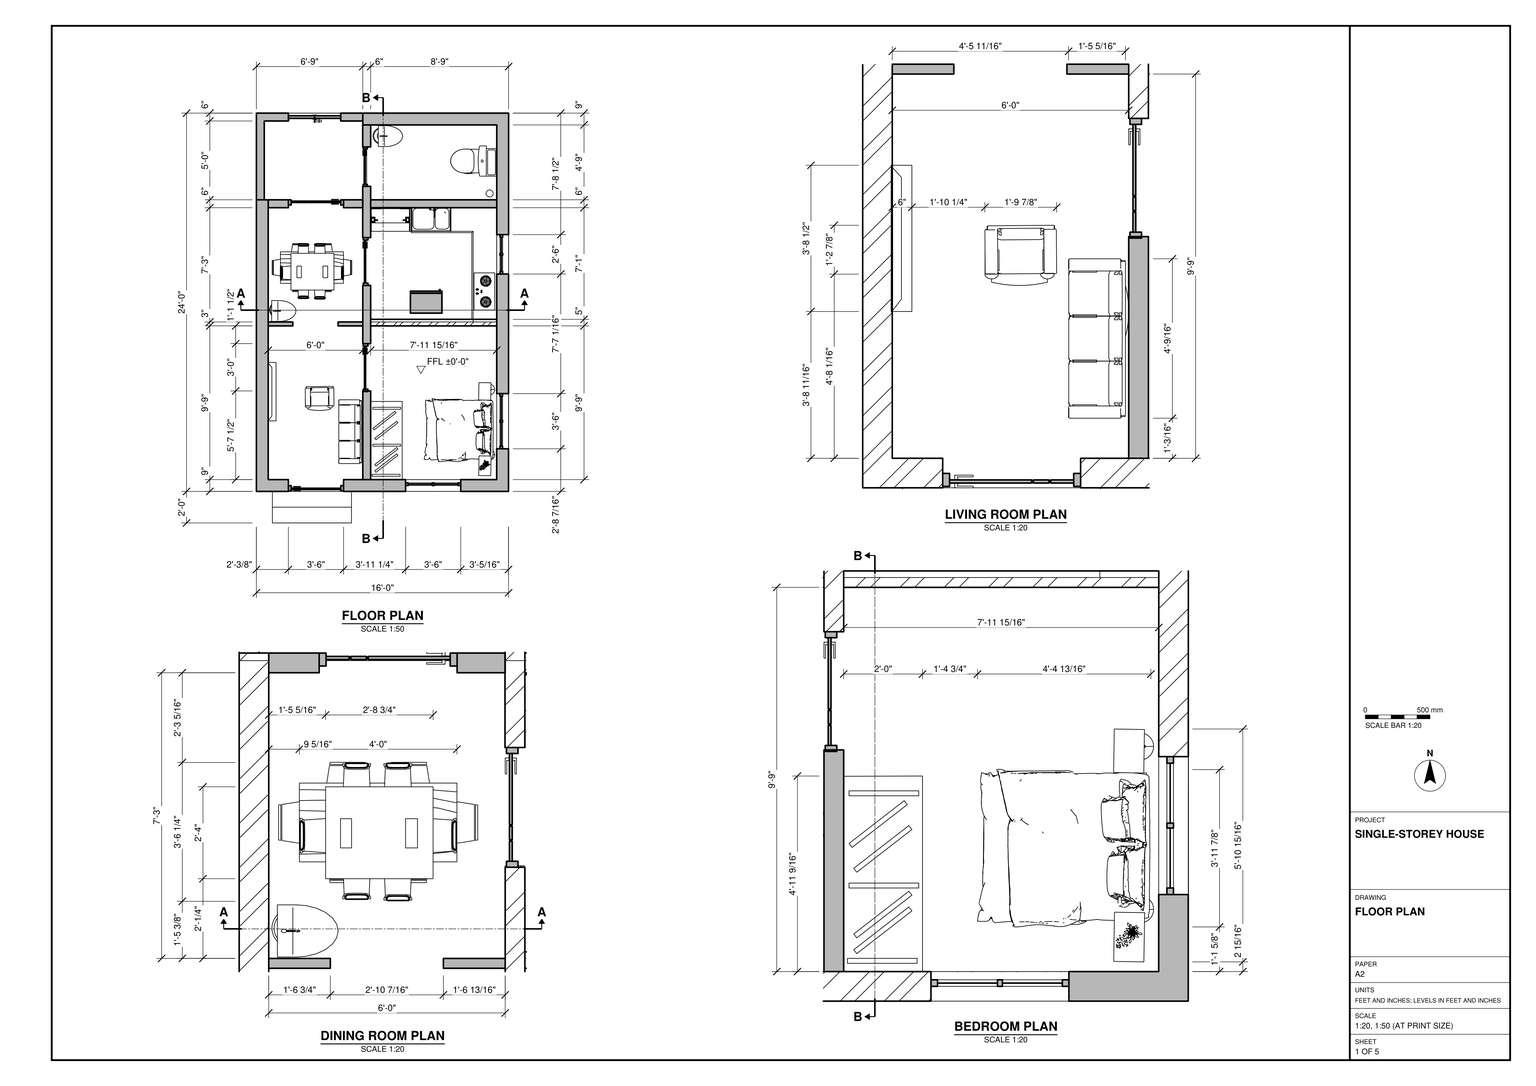
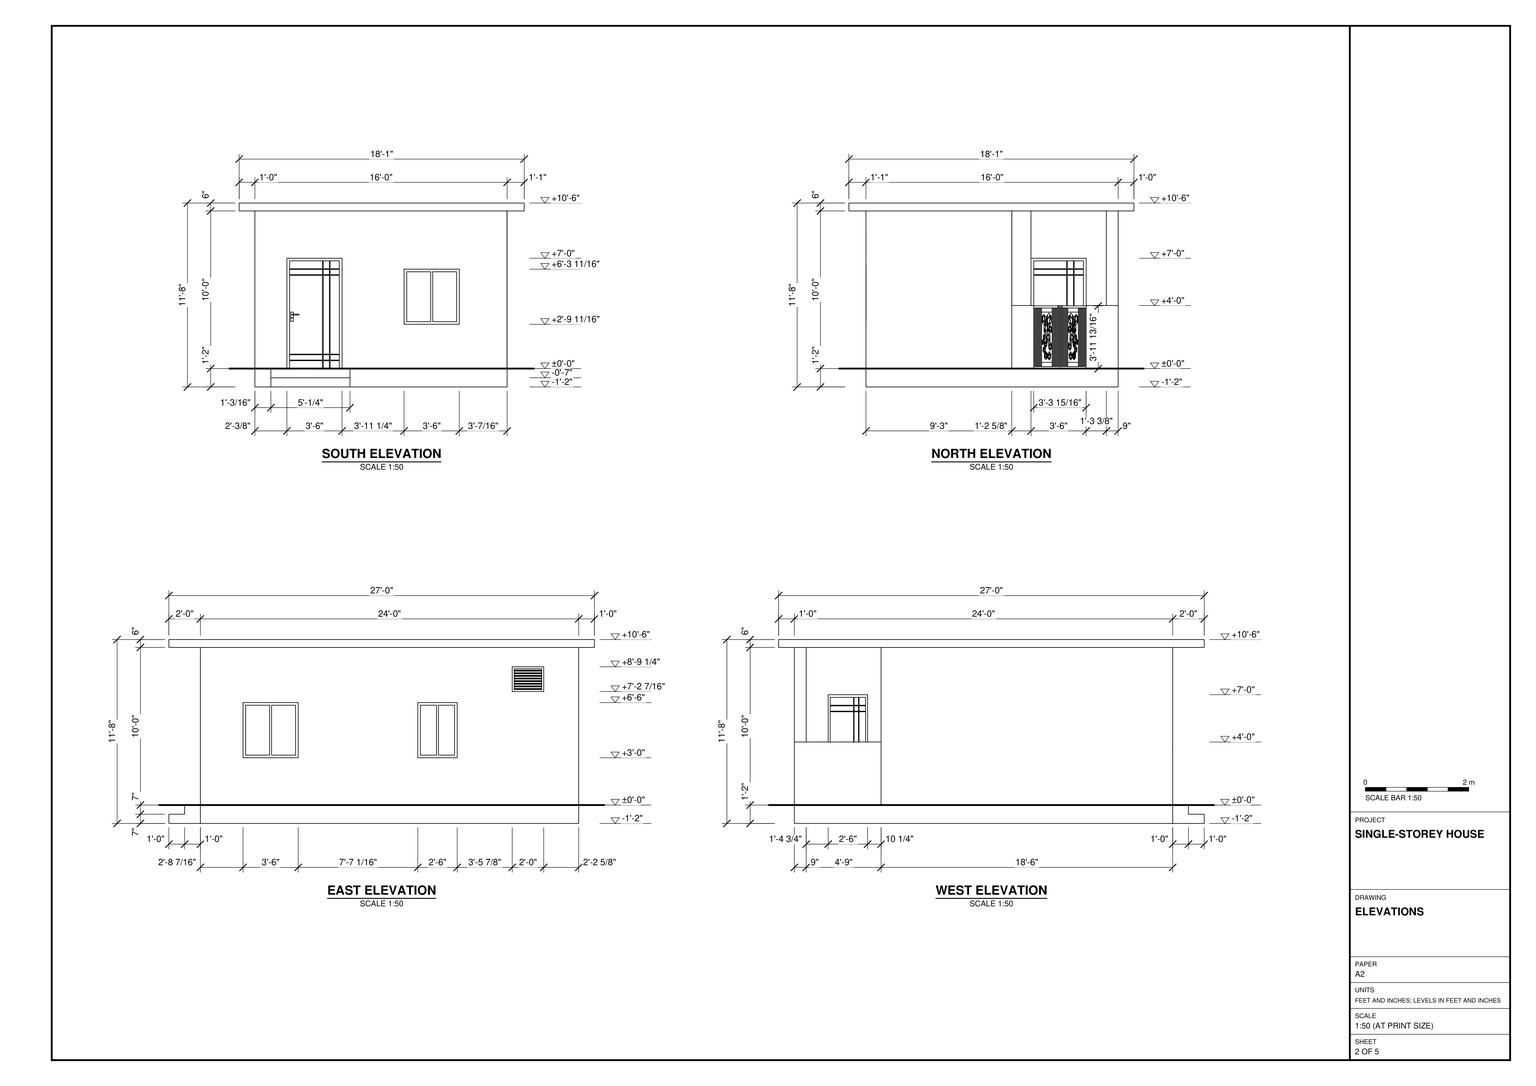
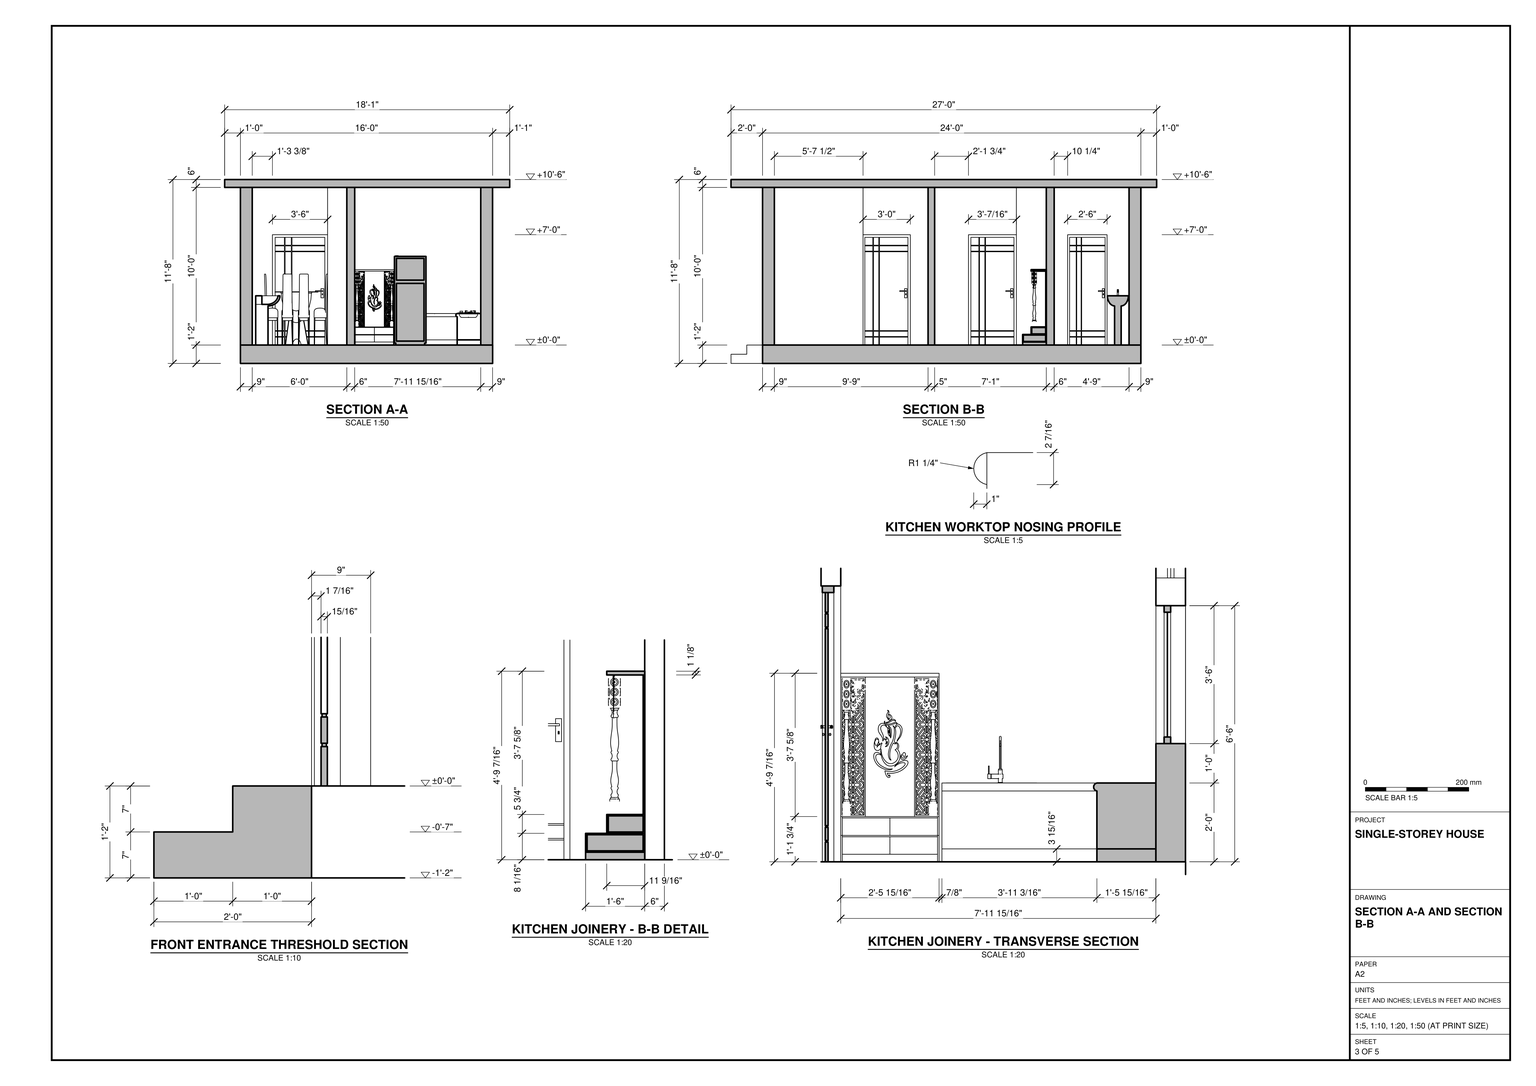
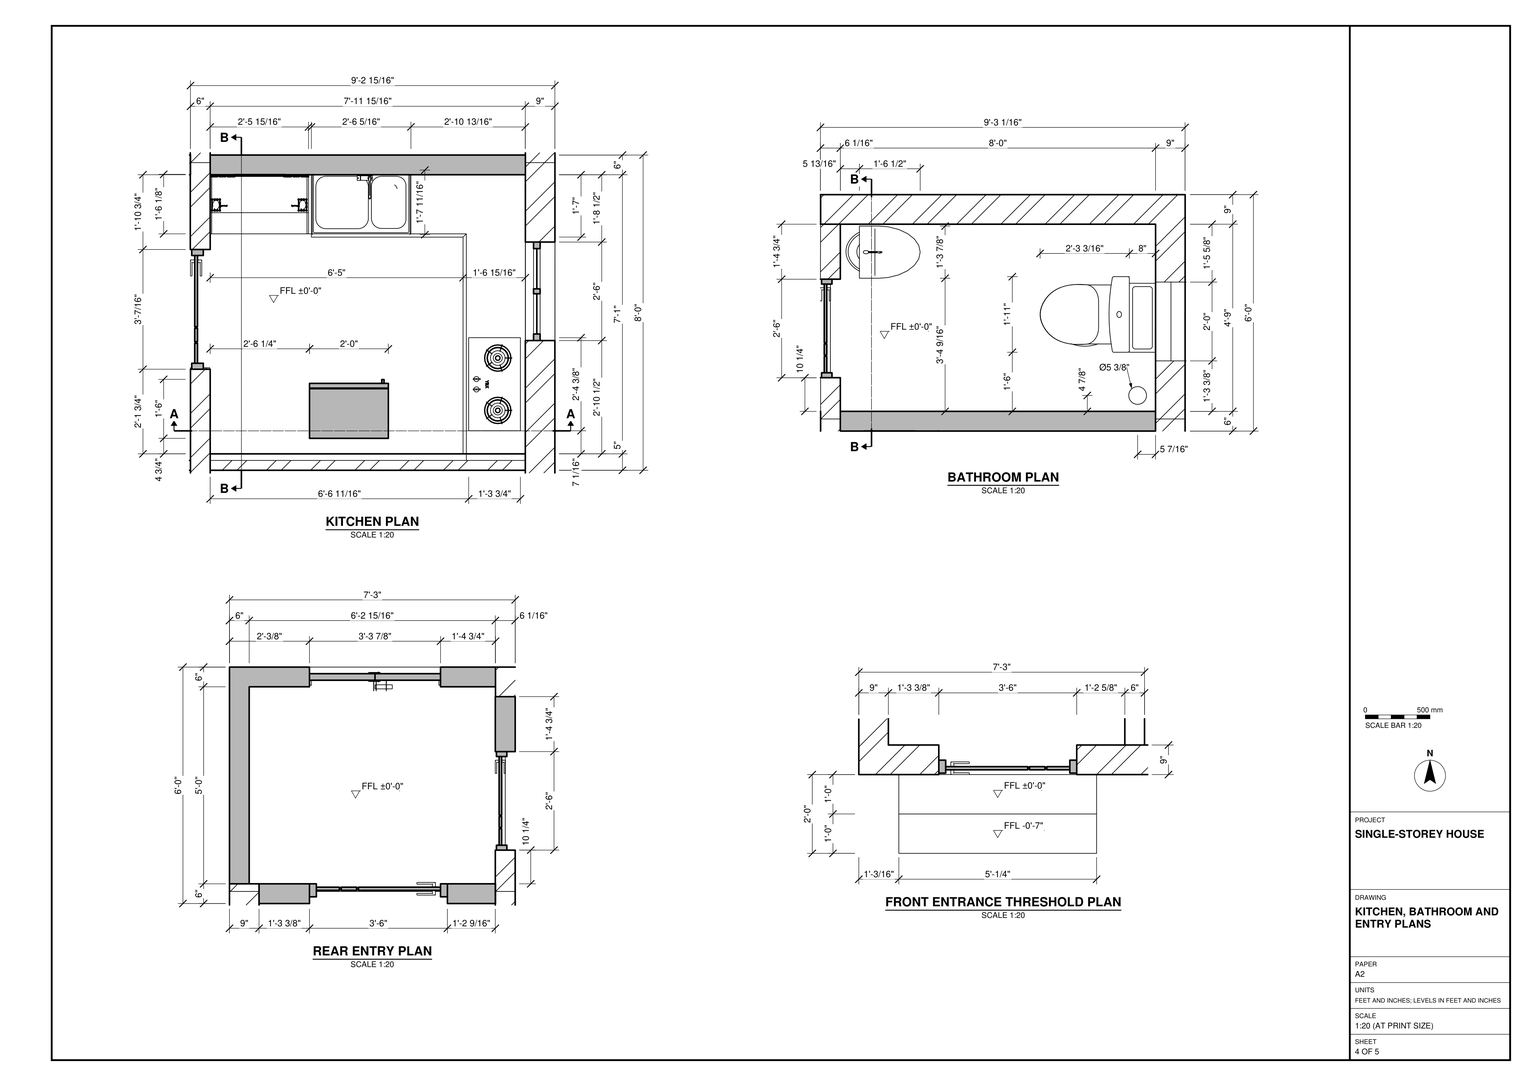
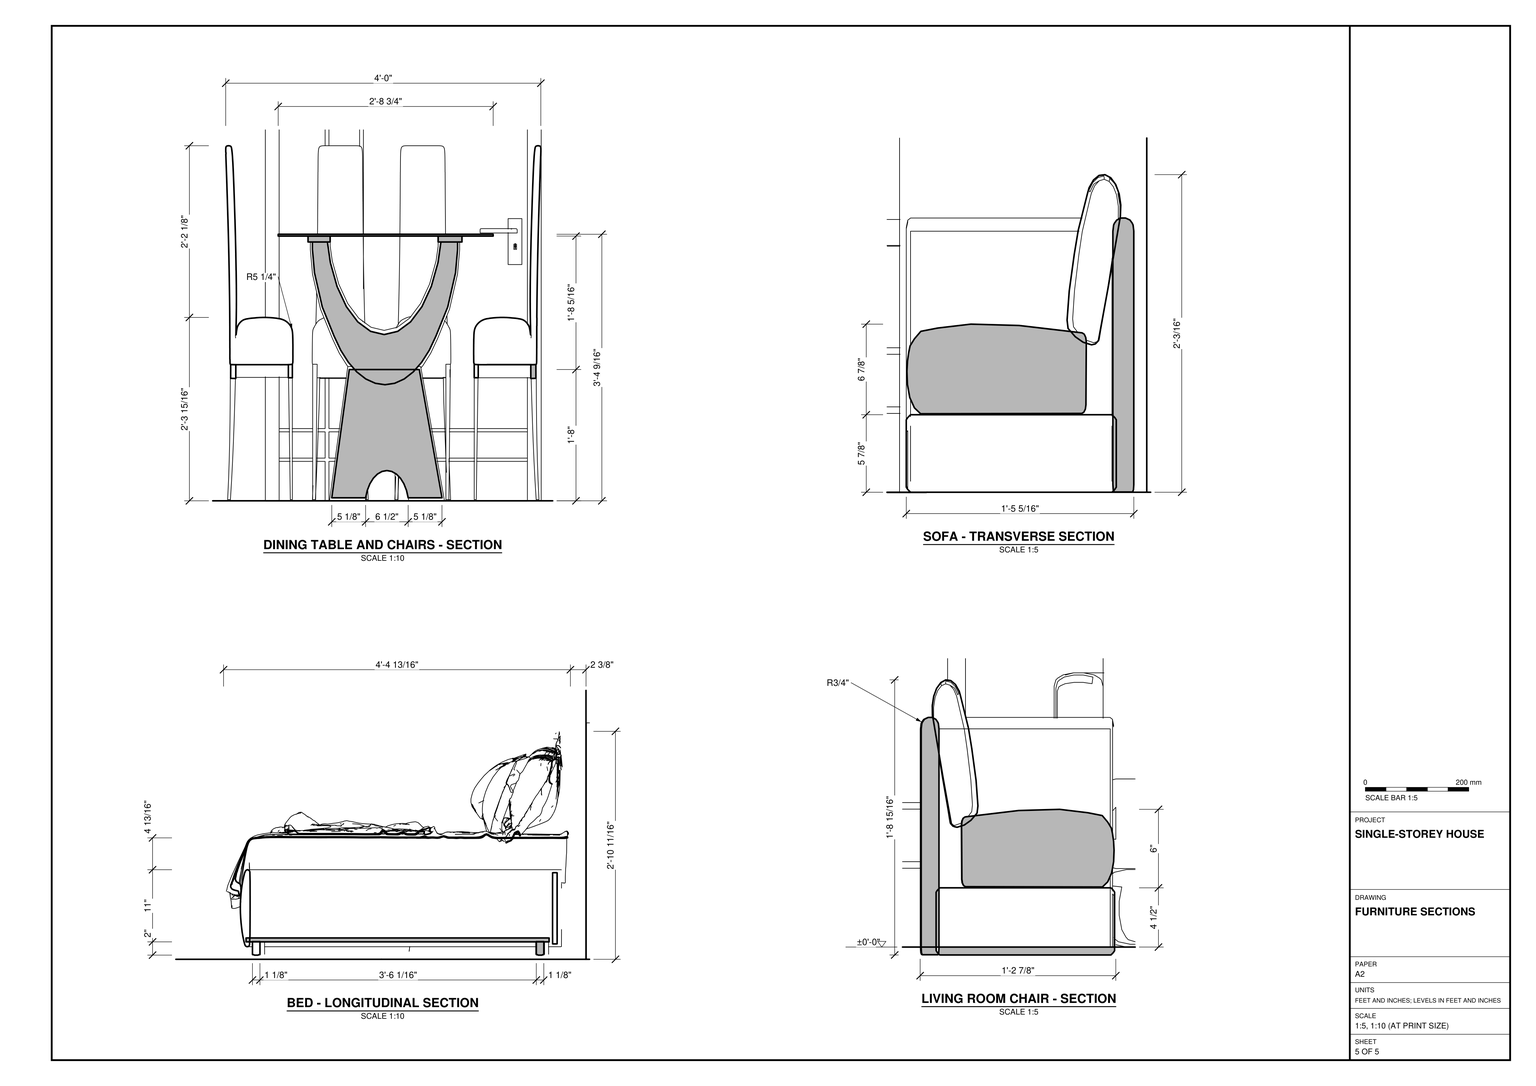
Build the single-storey house shown in task_files/diagram_01.pdf. Work in feet and inches. Set the finished ground floor at ±0'-0". The overall model is 18'-1" wide, 27'-0" long and 11'-8" high, including the raised base and projecting roof. The wall footprint is 16'-0" by 24'-0"; use this footprint, rather than the roof outline, to set out the rooms.

Model the floor slab, the stepped threshold at the south entrance and the flat roof slab with its unequal overhangs. Follow the plans and sections for wall thicknesses and door positions. Include the recessed area at the northwest corner, the framed windows and the high vent on the east elevation.

Place the living room and dining room along the west side. Arrange the sofa, chair and opposing wall unit as shown in the living room detail, and fit the dining table and chairs in the adjoining room. On the east side, model the bedroom with its bed, bedside units and storage, the kitchen with its fitted worktop and tall joinery unit, and the bathroom with its fixtures. Use the kitchen sections to shape the worktop edge and the base of the tall unit. Decor and loose items, including appliances, may be any suitable library components.

Keep the walls, slabs and roof as separate groups or components, and group each furniture or joinery piece separately. Use components for repeated parts. Save one SketchUp model as output_files/furnished_single_storey_house_with_a_stepped_entrance.skp.

# SketchUp Ruby script. Lengths in inches.
U = 1.inch
M = Sketchup.active_model
def pt(a) = Geom::Point3d.new(a.map { |v| v * U })
def face(e, loops, mat)
  f = e.add_face(loops[0].map { |a| pt(a) })
  loops[1..].each { |l| e.add_face(l.map { |a| pt(a) }).erase! }
  f.material = f.back_material = mat if mat
  f
end
# faces: each face lists its corners as indices into pts; further lists are holes
def faces(e, pts, list, mat = nil) = list.each { |f| face(e, (f[0].is_a?(Array) ? f : [f]).map { |l| l.map { |i| pts[i] } }, mat) }
# xy, xz, yz: faces in a plane at the given z, y or x. An outline is a flat list of corners, or four numbers for a rectangle; further outlines are holes
def ring(l) = l.size == 4 ? [[l[0], l[1]], [l[2], l[1]], [l[2], l[3]], [l[0], l[3]]] : l.each_slice(2).to_a
def flat(e, list, mat, &to3) = list.each { |f| face(e, (f[0].is_a?(Array) ? f : [f]).map { |l| ring(l).map { |u, v| to3.(u, v) } }, mat) }
def xy(e, z, list, mat = nil) = flat(e, list, mat) { |x, y| [x, y, z] }
def xz(e, y, list, mat = nil) = flat(e, list, mat) { |x, z| [x, y, z] }
def yz(e, x, list, mat = nil) = flat(e, list, mat) { |y, z| [x, y, z] }
def lines(e, pts, list) = list.each { |a, b| e.add_line(pt(pts[a]), pt(pts[b])) }
# prism: a flat outline (further loops are holes) pulled along v
def prism(e, loops, v, mat = nil)
  f = face(e, loops, mat); d = Geom::Vector3d.new(v.map { |x| x * U })
  f.pushpull(f.normal.samedirection?(d) ? d.length : -d.length)
end
def box(e, o, s, mat = nil) = prism(e, [[o, [o[0] + s[0], o[1], o[2]], [o[0] + s[0], o[1] + s[1], o[2]], [o[0], o[1] + s[1], o[2]]]], [0, 0, s[2]], mat)
def at(x, y, z, deg = 0) = Geom::Transformation.translation(pt([x, y, z])) * Geom::Transformation.rotation(ORIGIN, Z_AXIS, deg.degrees)
def axes(o, x, y, z) = Geom::Transformation.new([*x, 0, *y, 0, *z, 0, *pt(o).to_a, 1])
def part(name) = M.definitions.add(name)
# library, detail: a bought-in or finely detailed component or shape, given as its bounding box
def library(name, o, s) = part(name).tap { |d| box(d.entities, o, s) }
def detail(e, o, s) = box(e.add_group.entities, o, s)
def put(e, d, t, mat = nil) = e.add_instance(d, t).tap { |i| i.material = mat if mat }
def group(e, t, mat = nil) = e.add_group.tap { |g| g.transformation = t; g.material = mat if mat }.entities
root = M.entities
M.materials.add("0201 AP 9425 OUTDOOR PINK").color = [235, 192, 222]
M.materials.add("0241 AP 9602 Catmint Blossom-N").color = [202, 177, 218]
M.materials.add("0836 AP 7769 GREEN GLADE").color = [230, 225, 175]
M.materials.add("Colors In Model-1").color = [247, 231, 213]
M.materials.add("Picture1").color = [191, 175, 175]
M.materials.add("Picture2").color = [185, 162, 149]
M.materials.add("[Blacktop Old 02]").color = [143, 145, 145]
M.materials.add("[Carrera Marble]").color = [207, 207, 207]
M.materials.add("[Color B03]").color = [255, 140, 101]
M.materials.add("[Color H06]").color = [0, 204, 204]
M.materials.add("[Color L03]").color = [255, 101, 178]
M.materials.add("[Color M00]").color = [255, 255, 255]
M.materials.add("[Color M08]").color = [30, 30, 30]
M.materials.add("[Concrete Pavers Block Multi]").color = [124, 140, 145]
M.materials.add("[Field Rectangle Tile]").color = [196, 189, 179]
M.materials.add("[Formica Beige]").color = [211, 187, 149]
M.materials.add("[Marble Carrara Gold Floor Tile]").color = [225, 223, 217]
M.materials.add("[Metal Corrugated Shiny]1").color = [193, 193, 193]
M.materials.add("[Tile Border Travertine]").color = [160, 142, 112]
M.materials.add("[Translucent Glass Blue]").color = [100, 149, 237]
M.materials["[Translucent Glass Blue]"].alpha = 0.5
M.materials.add("[Wood Cherry Original]").color = [152, 86, 42]
M.materials.add("ft").color = [182, 168, 149]
c1 = library("Untitled",[0,0,0],[36,4.39,84])
c2 = library("Bedroom furniture set",[0,-4.61,0],[113.04,95.21,38.625])
c3 = part("Folded newspaper")
xy(c3.entities,0,[[0,2.76,135.04,80.9]],"Picture2")
xy(c3.entities,0.6,[[0,2.76,135.04,79.92]],"Colors In Model-1")
xy(c3.entities,1.45,[[0,2.8,135.04,79.875]],"Picture1")
xy(c3.entities,2.97,[[0,2.76,135.04,79.875]],"Colors In Model-1")
xy(c3.entities,3.82,[[0,2.76,135.04,79.92]],"Picture1")
xy(c3.entities,6.19,[[0,2.8,135.04,79.92]],"Picture1")
xy(c3.entities,7.04,[[0,2.04,135.04,2.76]],"Colors In Model-1")
xy(c3.entities,7.04,[[0,2.76,135.04,79.92],[0,79.92,24.36,80.26,127.45,80.26,135.04,79.92]],"Picture1")
xz(c3.entities,2.76,[[0,2.97,135.04,3.82]],"ft")
xz(c3.entities,79.92,[[0,6.19,135.04,7.04]],"Picture1")
yz(c3.entities,0,[[2.76,0.6,2.04,0.71,1.38,1.03,0.81,1.54,0.37,2.21,0.09,2.99,0,3.82,0.09,4.65,0.37,5.43,0.81,6.1,1.38,6.61,2.04,6.93,2.76,7.04,79.92,7.04,79.92,6.19,2.8,6.19,2.23,6.11,1.74,5.87,1.33,5.49,1,5,0.8,4.43,0.73,3.82,0.8,3.21,1,2.64,1.33,2.15,1.74,1.77,2.23,1.53,2.8,1.45,79.875,1.45,80.09,1.48,80.24,1.55,80.38,1.67,80.48,1.83,80.54,2.01,80.57,2.21,80.54,2.4,80.48,2.58,80.38,2.74,80.24,2.86,80.09,2.9375,79.875,2.97,2.76,2.97,2.76,3.82,79.92,3.82,80.28,3.76,80.61,3.6,80.9,3.35,81.11,3.01,81.25,2.625,81.3,2.21,81.25,1.79,81.11,1.4,80.9,1.07,80.61,0.8125,80.28,0.65,79.92,0.6]],"Picture1")
yz(c3.entities,135.04,[[2.76,0.6,79.92,0.6,80.28,0.65,80.61,0.8125,80.9,1.07,81.11,1.4,81.25,1.79,81.3,2.21,81.25,2.625,81.11,3.01,80.9,3.35,80.61,3.6,80.28,3.76,79.92,3.82,2.76,3.82,2.76,2.97,79.875,2.97,80.09,2.9375,80.24,2.86,80.38,2.74,80.48,2.58,80.54,2.4,80.57,2.21,80.54,2.01,80.48,1.83,80.38,1.67,80.24,1.55,80.09,1.48,79.875,1.45,2.8,1.45,2.23,1.53,1.74,1.77,1.33,2.15,1,2.64,0.8,3.21,0.73,3.82,0.8,4.43,1,5,1.33,5.49,1.74,5.87,2.23,6.11,2.8,6.19,79.92,6.19,79.92,7.04,2.76,7.04,2.04,6.93,1.38,6.61,0.81,6.1,0.37,5.43,0.09,4.65,0,3.82,0.09,2.99,0.37,2.21,0.81,1.54,1.38,1.03,2.04,0.71]],"Picture1")
p = [[0,2.04,0.71],[0,2.76,0.6],[135.04,2.76,0.6],[135.04,2.04,0.71],[0,79.92,0.6],[0,80.28,0.65],
  [135.04,80.28,0.65],[135.04,79.92,0.6],[0,1.38,1.03],[135.04,1.38,1.03],[0,80.61,0.8125],[135.04,80.61,0.8125],
  [0,80.9,1.07],[135.04,80.9,1.07],[0,0.81,1.54],[135.04,0.81,1.54],[0,81.11,1.4],[135.04,81.11,1.4],
  [0,2.8,1.45],[0,2.23,1.53],[135.04,2.23,1.53],[135.04,2.8,1.45],[0,80.09,1.48],[0,79.875,1.45],
  [135.04,79.875,1.45],[135.04,80.09,1.48],[0,81.25,1.79],[135.04,81.25,1.79],[0,0.37,2.21],[135.04,0.37,2.21],
  [0,1.74,1.77],[135.04,1.74,1.77],[0,80.24,1.55],[135.04,80.24,1.55],[0,80.38,1.67],[135.04,80.38,1.67],
  [0,80.48,1.83],[135.04,80.48,1.83],[0,1.33,2.15],[135.04,1.33,2.15],[0,80.54,2.01],[135.04,80.54,2.01],
  [0,81.3,2.21],[135.04,81.3,2.21],[0,80.57,2.21],[135.04,80.57,2.21],[0,1,2.64],[135.04,1,2.64],
  [0,0.09,2.99],[135.04,0.09,2.99],[0,80.54,2.4],[135.04,80.54,2.4],[0,81.25,2.625],[135.04,81.25,2.625],
  [0,80.48,2.58],[135.04,80.48,2.58],[0,0.8,3.21],[135.04,0.8,3.21],[0,80.38,2.74],[135.04,80.38,2.74],
  [0,81.11,3.01],[135.04,81.11,3.01],[0,80.24,2.86],[135.04,80.24,2.86],[0,79.875,2.97],[0,80.09,2.9375],
  [135.04,80.09,2.9375],[135.04,79.875,2.97],[0,0,3.82],[135.04,0,3.82],[0,80.9,3.35],[135.04,80.9,3.35],
  [0,0.73,3.82],[135.04,0.73,3.82],[0,80.61,3.6],[135.04,80.61,3.6],[0,80.28,3.76],[135.04,80.28,3.76],
  [0,0.09,4.65],[135.04,0.09,4.65],[0,0.8,4.43],[135.04,0.8,4.43],[0,79.92,3.82],[135.04,79.92,3.82],
  [0,1,5],[135.04,1,5],[0,0.37,5.43],[135.04,0.37,5.43],[0,1.33,5.49],[135.04,1.33,5.49],
  [0,0.81,6.1],[135.04,0.81,6.1],[0,1.74,5.87],[135.04,1.74,5.87],[0,2.23,6.11],[135.04,2.23,6.11],
  [0,1.38,6.61],[135.04,1.38,6.61],[0,2.8,6.19],[135.04,2.8,6.19],[0,2.04,6.93],[135.04,2.04,6.93],
  [0,2.76,7.04],[135.04,2.76,7.04]]
faces(c3.entities,p,[[0,1,2,3],[4,5,6,7],[8,0,3,9],[5,10,11,6],[10,12,13,11],[14,8,9,15],[12,16,17,13],[18,19,20,21],
  [16,26,27,17],[28,14,15,29],[19,30,31,20],[30,38,39,31],[26,42,43,27],[38,46,47,39],[48,28,29,49],[42,52,53,43],
  [46,56,57,47],[52,60,61,53],[68,48,49,69],[60,70,71,61],[56,72,73,57],[70,74,75,71],[74,76,77,75],[78,68,69,79],
  [72,80,81,73],[76,82,83,77],[80,84,85,81],[86,78,79,87],[84,88,89,85],[90,86,87,91],[88,92,93,89],[92,94,95,93],
  [96,90,91,97],[94,98,99,95],[100,96,97,101],[102,100,101,103]],"Picture1")
faces(c3.entities,p,[[22,23,24,25],[32,22,25,33],[34,32,33,35],[36,34,35,37],[40,36,37,41],[44,40,41,45],[50,44,45,51],[54,50,51,55],
  [58,54,55,59],[62,58,59,63],[64,65,66,67],[65,62,63,66]],"ft")
c4 = part("News Paper")
put(c4.entities,c3,at(-7.68,7.68,0))
c5 = part("Sofa - Roundback Loveseat 5 ft.")
p = [[0,-15.44,0],[0,11,0],[-24,-17,0],[-30,-17,0],[-30,9,0],[-24,5.53,0],
  [-24,-15.44,0],[24,-15.44,0],[-24,3.62,0],[24,3.62,0],[24,5.53,0],[20.76,6.96,0],
  [17.43,8.1875,0],[14.03,9.19,0],[10.57,9.98,0],[7.07,10.55,0],[3.54,10.89,0],[-3.54,10.89,0],
  [-7.07,10.55,0],[-10.57,9.98,0],[-14.03,9.19,0],[-17.43,8.1875,0],[-20.76,6.96,0],[30,9,0],
  [26.53,10.84,0],[22.96,12.46,0],[19.28,13.83,0],[15.52,14.97,0],[11.7,15.85,0],[7.83,16.49,0],
  [3.92,16.87,0],[0,17,0],[-3.92,16.87,0],[-7.83,16.49,0],[-11.7,15.85,0],[-15.52,14.97,0],
  [-19.28,13.83,0],[-22.96,12.46,0],[-26.53,10.84,0],[30,-17,0],[24,-17,0]]
lines(c5.entities,p,[[0,1],[2,3],[3,4],[2,5],[6,7],[8,9],[10,11],[11,12],[12,13],[13,14],[14,15],[15,16],
  [16,1],[1,17],[17,18],[18,19],[19,20],[20,21],[21,22],[22,5],[23,24],[24,25],[25,26],[26,27],
  [27,28],[28,29],[29,30],[30,31],[31,32],[32,33],[33,34],[34,35],[35,36],[36,37],[37,38],[38,4],
  [23,39],[39,40],[40,10]])
c6 = library("Lamp - Table",[-7,-7,0],[14,14,0.01])
c7 = library("Chair - Desk",[-10.5,-8.5,0],[21,17,0.01])
c8 = library("Dining Set - 36 x 72 in.",[-45.5,-27.5,0],[91,55,0.01])
c9 = library("Sink - Oval top",[-12.23,-10.02,0],[24.46,20.04,0.01])
c10 = part("tv unit")
p = [[-5.32,37.84,0],[5.41,37.84,0],[5.41,-37.53,0],[-5.32,-37.53,0],[-5.41,37.625,0],[0,31.58,0],
  [0,-31.12,0],[-5.15,-37.84,0]]
lines(c10.entities,p,[[0,1],[1,2],[2,3],[3,0],[4,5],[5,6],[6,7]])
c11 = library("Toilet - top",[-10.5,-16.5,0],[21,33,0.01])
c12 = part("MY HOUSE PLAN.dwg")
xy(c12.entities,0,[[81,9,87,76.5]])
xy(c12.entities,120,[[81,9,87,76.5]],"[Color M00]")
xz(c12.entities,9,[[81,0,81.4,120],[81.4,0,85.89,120],[85.89,0,87,120]])
xz(c12.entities,76.5,[[81,0,87,120]])
yz(c12.entities,81,[[9,0,76.5,120]],"[Color H06]")
yz(c12.entities,87,[[9,0,76.5,120]],"0201 AP 9425 OUTDOOR PINK")
# 335 loose lines left out
put(c12.entities,c5,axes([72.23,53.81,0],[0,-0.51611,0],[0.51611,0,0],[0,0,0.51611]))
put(c12.entities,c6,axes([177.25,77.5625,0],[0.58792,0,0],[0,0.58792,0],[0,0,0.58792]))
put(c12.entities,c6,axes([177.25,27.94,0],[0.58792,0,0],[0,0.58792,0],[0,0,0.58792]))
put(c12.entities,c7,at(47.75,70.12,0))
put(c12.entities,c8,axes([42.3125,170.4,0],[0.66638,0,0],[0,0.66638,0],[0,0,0.66638]))
put(c12.entities,c9,axes([18.39,138.16,0],[0.68707,0,0],[0,0.68707,0],[0,0,0.68707]))
put(c12.entities,c10,axes([11.79,75.87,0],[0.5907,0,0],[0,0.5907,0],[0,0,0.5907]))
put(c12.entities,c9,axes([97.13,270.59,0],[0.68707,0,0],[0,0.68707,0],[0,0,0.68707]))
put(c12.entities,c11,at(166.5,250.5,0,-90))
c13 = library("2-EVIER M80 CLC2",[-15.14,-9.87,-6.7],[30.32,19.69,21.06])
c14 = library("Gas stove",[25.14,27.93,-3.15],[28.35,15.74,5.16])
c15 = library("Household shrine",[0,0,0],[62.99,27.68,98.43])
c16 = library("canapele",[-158.28,104.78,-0.6],[42.82,58.76,24.78])
c17 = library("Gate_Lasercut_10ftx6ft_Kalil",[-0.15,-3.25,-0.15],[120,5.625,60.3])
c18 = part("Refridgerator")
g1 = group(c18.entities,at(117.47,72.48,0,-90))
g2 = group(g1,at(21.25,0,2.03))
g3 = group(g2,at(0,1.5,47.41))
xy(g3,-0.5,[[0,-1.5,2,22.5]],"[Metal Corrugated Shiny]1")
xy(g3,18.0625,[[0,-1.5,2,22.5]],"[Metal Corrugated Shiny]1")
xz(g3,-1.5,[[0,-0.5,2,18.0625]],"[Metal Corrugated Shiny]1")
xz(g3,22.5,[[0,-0.5,2,18.0625]],"[Metal Corrugated Shiny]1")
yz(g3,0,[[-1.5,-0.5,22.5,18.0625]],"[Metal Corrugated Shiny]1")
yz(g3,2,[[15.47,13.9,19.65,15.65]],"[Color M08]")
yz(g3,2,[[[-1.5,-0.5,22.5,18.0625],[15.47,13.9,19.65,15.65]]],"[Metal Corrugated Shiny]1")
g4 = group(g2,at(0,1.5,1.25))
box(g4,[0,-1.5,-1.25],[2,24,46.41],"[Metal Corrugated Shiny]1")
g5 = group(g2,at(1.125,1.3125,47.66))
prism(g5,[[[0.9,0.6875,10.53],[0.9,0.6875,14],[1.24,0.6875,12.86],[1.53,0.6875,11.71],[1.8,0.6875,10.55],[2.02,0.6875,9.39],[2.21,0.6875,8.22],[2.36,0.6875,7.05],[2.47,0.6875,5.88],[2.55,0.6875,4.7],[2.59,0.6875,3.53],[2.59,0.6875,2.35],[2.55,0.6875,1.18],[2.48,0.6875,0],[0.9,0.6875,0],[0.9,0.6875,0.75],[1.58,0.6875,0.75],[1.62,0.6875,0.75],[1.65,0.6875,1.18],[1.6875,0.6875,2.35],[1.6875,0.6875,3.53],[1.65,0.6875,4.7],[1.57,0.6875,5.88],[1.46,0.6875,7.05],[1.31,0.6875,8.22],[1.12,0.6875,9.39]]],[0,-0.6875,0],"[Metal Corrugated Shiny]1")
# 4 loose lines left out
g6 = group(g2,at(1.125,2,45.66))
prism(g6,[[[0.9,-0.6875,-10.53],[0.9,-0.6875,-14],[1.24,-0.6875,-12.86],[1.53,-0.6875,-11.71],[1.8,-0.6875,-10.55],[2.02,-0.6875,-9.39],[2.21,-0.6875,-8.22],[2.36,-0.6875,-7.05],[2.47,-0.6875,-5.88],[2.55,-0.6875,-4.7],[2.59,-0.6875,-3.53],[2.59,-0.6875,-2.35],[2.55,-0.6875,-1.18],[2.48,-0.6875,0],[0.9,-0.6875,0],[0.9,-0.6875,-0.75],[1.58,-0.6875,-0.75],[1.62,-0.6875,-0.75],[1.65,-0.6875,-1.18],[1.6875,-0.6875,-2.35],[1.6875,-0.6875,-3.53],[1.65,-0.6875,-4.7],[1.57,-0.6875,-5.88],[1.46,-0.6875,-7.05],[1.31,-0.6875,-8.22],[1.12,-0.6875,-9.39]]],[0,0.6875,0],"[Metal Corrugated Shiny]1")
# 4 loose lines left out
g7 = group(g1,at(0,0,0))
g8 = group(g7,at(20.8125,-2.49,68.0625))
xy(g8,-0.5,[[-1.6875,23.55,-1.97,23.58,-2.24,23.69,-2.46,23.87,-2.64,24.09,-2.75,24.36,-2.78,24.64,-2.75,24.93,-2.64,25.19,-2.46,25.42,-2.24,25.59,-1.97,25.7,-1.6875,25.74,0.9,25.74,1.1875,25.7,1.45,25.59,1.68,25.42,1.85,25.19,1.96,24.93,2,24.64,1.96,24.36,1.85,24.09,1.68,23.87,1.45,23.69,1.1875,23.58,0.9,23.55]],"[Metal Corrugated Shiny]1")
xy(g8,0,[[-1.6875,23.55,0.9,23.55,0.9,25.74,-1.6875,25.74,-1.97,25.7,-2.24,25.59,-2.46,25.42,-2.64,25.19,-2.75,24.93,-2.78,24.64,-2.75,24.36,-2.64,24.09,-2.46,23.87,-2.24,23.69,-1.97,23.58],[0.9,23.55,1.1875,23.58,1.45,23.69,1.68,23.87,1.85,24.09,1.96,24.36,2,24.64,1.96,24.93,1.85,25.19,1.68,25.42,1.45,25.59,1.1875,25.7,0.9,25.74]],"[Metal Corrugated Shiny]1")
xz(g8,23.55,[[-1.6875,-0.5,0.9,0]],"[Metal Corrugated Shiny]1")
xz(g8,25.74,[[-1.6875,-0.5,0.9,0]],"[Metal Corrugated Shiny]1")
p = [[-1.6875,23.55,0],[-1.97,23.58,0],[-1.97,23.58,-0.5],[-1.6875,23.55,-0.5],[1.1875,23.58,0],[0.9,23.55,0],
  [0.9,23.55,-0.5],[1.1875,23.58,-0.5],[-2.24,23.69,0],[-2.24,23.69,-0.5],[1.45,23.69,0],[1.45,23.69,-0.5],
  [-2.46,23.87,0],[-2.46,23.87,-0.5],[1.68,23.87,0],[1.68,23.87,-0.5],[-2.64,24.09,0],[-2.64,24.09,-0.5],
  [1.85,24.09,0],[1.85,24.09,-0.5],[-2.75,24.36,0],[-2.75,24.36,-0.5],[1.96,24.36,0],[1.96,24.36,-0.5],
  [-2.78,24.64,0],[-2.78,24.64,-0.5],[2,24.64,0],[2,24.64,-0.5],[-2.75,24.93,0],[-2.75,24.93,-0.5],
  [1.96,24.93,0],[1.96,24.93,-0.5],[-2.64,25.19,0],[-2.64,25.19,-0.5],[1.85,25.19,0],[1.85,25.19,-0.5],
  [-2.46,25.42,0],[-2.46,25.42,-0.5],[1.68,25.42,0],[1.68,25.42,-0.5],[-2.24,25.59,0],[-2.24,25.59,-0.5],
  [1.45,25.59,0],[1.45,25.59,-0.5],[-1.97,25.7,0],[-1.97,25.7,-0.5],[1.1875,25.7,0],[1.1875,25.7,-0.5],
  [-1.6875,25.74,0],[-1.6875,25.74,-0.5],[0.9,25.74,0],[0.9,25.74,-0.5]]
faces(g8,p,[[0,1,2,3],[4,5,6,7],[1,8,9,2],[10,4,7,11],[8,12,13,9],[14,10,11,15],[12,16,17,13],[18,14,15,19],
  [16,20,21,17],[22,18,19,23],[20,24,25,21],[26,22,23,27],[24,28,29,25],[30,26,27,31],[28,32,33,29],[34,30,31,35],
  [32,36,37,33],[38,34,35,39],[36,40,41,37],[42,38,39,43],[40,44,45,41],[46,42,43,47],[44,48,49,45],[50,46,47,51]],"[Metal Corrugated Shiny]1")
g9 = group(g7,at(0,0,0))
xy(g9,0,[[1,1,20,23]],"[Metal Corrugated Shiny]1")
xy(g9,1.5,[[[0,0,21,24],[1,1,20,23]]],"[Metal Corrugated Shiny]1")
xy(g9,3,[[2,1.5,21,22.5]],"[Metal Corrugated Shiny]1")
xy(g9,46.9375,[[2,1.5,21,22.5]],"[Metal Corrugated Shiny]1")
xy(g9,49.4375,[[2,1.5,21,22.5]],"[Metal Corrugated Shiny]1")
xy(g9,66,[[2,1.5,21,22.5]],"[Metal Corrugated Shiny]1")
xy(g9,67.5,[[0,0,21,24]],"[Metal Corrugated Shiny]1")
xz(g9,0,[[0,1.5,21,67.5]],"[Metal Corrugated Shiny]1")
xz(g9,1,[[1,0,20,1.5]],"[Metal Corrugated Shiny]1")
xz(g9,1.5,[[2,3,21,46.9375],[2,49.4375,21,66]],"[Metal Corrugated Shiny]1")
xz(g9,22.5,[[2,3,21,46.9375],[2,49.4375,21,66]],"[Metal Corrugated Shiny]1")
xz(g9,23,[[1,0,20,1.5]],"[Metal Corrugated Shiny]1")
xz(g9,24,[[0,1.5,21,67.5]],"[Metal Corrugated Shiny]1")
yz(g9,0,[[0,1.5,24,67.5]],"[Metal Corrugated Shiny]1")
yz(g9,1,[[1,0,23,1.5]],"[Metal Corrugated Shiny]1")
yz(g9,2,[[1.5,3,22.5,46.9375],[1.5,49.4375,22.5,66]],"[Metal Corrugated Shiny]1")
yz(g9,20,[[1,0,23,1.5]],"[Metal Corrugated Shiny]1")
yz(g9,21,[[[0,1.5,24,67.5],[1.5,3,22.5,46.9375],[1.5,49.4375,22.5,66]]],"[Metal Corrugated Shiny]1")
c19 = library("Mesa+de+Jantar+Clean-Ouro",[18.32,209.12,6],[46.68,36.13,54.07])
c20 = library("Vask",[0,0,0],[10.95,18.9,37.68])
c21 = library("CS300DRT",[0,0,0],[27.18,17.85,30.31])
c22 = part("Group19\#1")
xy(c22.entities,0,[[87,126,182.95,131]])
xy(c22.entities,120,[[87,126,182.95,131]],"[Color B03]")
xz(c22.entities,126,[[87,0,182.95,120]],"0201 AP 9425 OUTDOOR PINK")
xz(c22.entities,131,[[87,0,182.95,120]],"[Color B03]")
yz(c22.entities,87,[[126,0,131,120]])
c23 = part("Group16\#1")
xy(c23.entities,0,[[87,216,182.98,222]])
xy(c23.entities,120,[[87,216,182.98,222]])
xz(c23.entities,216,[[87,0,182.98,120]],"[Color B03]")
xz(c23.entities,222,[[87,0,182.98,120]],"[Tile Border Travertine]")
yz(c23.entities,87,[[216,0,222,120]])
yz(c23.entities,182.98,[[216,0,222,120]])
c24 = part("Group18\#1")
xy(c24.entities,0,[[66.36,216,81,222]])
xy(c24.entities,120,[[66.36,216,81,222]])
xz(c24.entities,216,[[66.36,0,81,120]])
xz(c24.entities,222,[[66.36,0,81,120]],"[Field Rectangle Tile]")
yz(c24.entities,66.36,[[216,0,222,120]])
yz(c24.entities,81,[[216,0,222,120]])
c25 = part("Difference\#1")
xy(c25.entities,0,[[0,-69.03,6.06,-30],[0,0,6.06,16.74]],"[Formica Beige]")
xy(c25.entities,84,[[0,-30,6.06,0]],"[Formica Beige]")
xy(c25.entities,120,[[0,-69.03,6.06,16.74]],"[Formica Beige]")
xz(c25.entities,-69.03,[[0,0,6.06,120]],"[Formica Beige]")
xz(c25.entities,-30,[[0,0,6.06,84]],"[Formica Beige]")
xz(c25.entities,0,[[0,0,6.06,84]],"[Formica Beige]")
xz(c25.entities,16.74,[[0,0,6.06,120]],"[Formica Beige]")
yz(c25.entities,0,[[-69.03,0,-69.03,120,16.74,120,16.74,0,0,0,0,84,-30,84,-30,0]],"[Color H06]")
yz(c25.entities,6.06,[[-69.03,0,-30,0,-30,84,0,84,0,0,16.74,0,16.74,120,-69.03,120]],"0201 AP 9425 OUTDOOR PINK")
c26 = part("Difference\#2")
xy(c26.entities,0,[[81,112.5,87,156.77]])
xy(c26.entities,84,[[81,76.5,87,112.5],[81,156.77,87,193.23]])
xy(c26.entities,120,[[81,76.5,87,193.23]])
xz(c26.entities,76.5,[[81,84,87,120]])
xz(c26.entities,112.5,[[81,0,87,84]])
xz(c26.entities,156.77,[[81,0,87,84]])
xz(c26.entities,193.23,[[81,84,87,120]])
yz(c26.entities,81,[[112.5,0,112.5,84,76.5,84,76.5,120,193.23,120,193.23,84,156.77,84,156.77,0]],"[Color H06]")
yz(c26.entities,87,[[112.5,0,156.77,0,156.77,84,193.23,84,193.23,120,76.5,120,76.5,84,112.5,84]],"0201 AP 9425 OUTDOOR PINK")
c27 = part("Difference\#3")
xy(c27.entities,0,[[0,0,0,222,9,222,9,9,24.36,9,24.36,0],[66.36,0,66.36,9,182.91,9,183,279,81,279,81,288,192,288,191.91,0]])
xy(c27.entities,33.69,[[113.58,0,155.58,9]],"0201 AP 9425 OUTDOOR PINK")
xy(c27.entities,36,[[182.92,32.46,191.92,32.46,191.93,74.46,182.93,74.46],[182.96,165.5,191.96,165.5,191.97,195.5,182.97,195.5]],"0201 AP 9425 OUTDOOR PINK")
xy(c27.entities,75.69,[[113.58,0,155.58,9]])
xy(c27.entities,78,[[182.92,32.46,182.93,74.46,191.93,74.46,191.92,32.46],[182.96,165.5,182.97,195.5,191.97,195.5,191.96,165.5]])
xy(c27.entities,84,[[24.36,0,66.36,9]])
xy(c27.entities,86.4375,[[182.98,237.375,191.98,237.375,191.99,261.375,182.99,261.375]])
xy(c27.entities,105.25,[[182.98,237.375,182.99,261.375,191.99,261.375,191.98,237.375]])
xy(c27.entities,120,[[0,0,191.91,0,192,288,81,288,81,279,183,279,182.91,9,9,9,9,222,0,222]])
xz(c27.entities,0,[[[0,0,24.36,0,24.36,84,66.36,84,66.36,0,191.91,0,191.91,120,0,120],[113.58,33.69,155.58,75.69]]])
xz(c27.entities,9,[[[9,0,9,120,182.91,120,182.91,0,66.36,0,66.36,84,24.36,84,24.36,0],[113.58,33.69,155.58,75.69]]],"0201 AP 9425 OUTDOOR PINK")
xz(c27.entities,32.46,[[182.92,36,191.92,78]])
xz(c27.entities,74.46,[[182.93,36,191.93,78]])
xz(c27.entities,165.5,[[182.96,36,191.96,78]],"0201 AP 9425 OUTDOOR PINK")
xz(c27.entities,195.5,[[182.97,36,191.97,78]],"0201 AP 9425 OUTDOOR PINK")
xz(c27.entities,222,[[0,0,9,120]])
xz(c27.entities,237.375,[[182.98,86.4375,191.98,105.25]])
xz(c27.entities,261.375,[[182.99,86.4375,191.99,105.25]])
xz(c27.entities,279,[[81,0,183,120]],"[Tile Border Travertine]")
xz(c27.entities,288,[[81,0,192,120]])
yz(c27.entities,0,[[0,0,222,120]])
yz(c27.entities,9,[[9,0,222,120]],"[Color H06]")
yz(c27.entities,24.36,[[0,0,9,84]])
yz(c27.entities,66.36,[[0,0,9,84]])
yz(c27.entities,81,[[279,0,288,120]])
yz(c27.entities,113.58,[[0,33.69,9,75.69]])
yz(c27.entities,155.58,[[0,33.69,9,75.69]])
# 1 loose lines left out
p = [[191.91,0,120],[191.91,0,0],[192,288,0],[192,288,120],[191.93,74.46,36],[191.92,32.46,36],
  [191.92,32.46,78],[191.93,74.46,78],[191.96,165.5,36],[191.96,165.5,78],[191.97,195.5,78],[191.97,195.5,36],
  [191.98,237.375,105.25],[191.99,261.375,105.25],[191.99,261.375,86.4375],[191.98,237.375,86.4375],[182.91,9,0],[182.91,9,120],
  [183,279,120],[183,279,0],[182.92,32.46,36],[182.93,74.46,36],[182.93,74.46,78],[182.92,32.46,78],
  [182.97,195.5,36],[182.97,195.5,78],[182.96,165.5,78],[182.96,165.5,36],[182.99,261.375,105.25],[182.98,237.375,105.25],
  [182.98,237.375,86.4375],[182.99,261.375,86.4375]]
faces(c27.entities,p,[[[0,1,2,3],[4,5,6,7],[8,9,10,11],[12,13,14,15]]])
faces(c27.entities,p,[[[16,17,18,19],[20,21,22,23],[24,25,26,27],[28,29,30,31]]],"0201 AP 9425 OUTDOOR PINK")
c28 = part("Group25\#2")
xy(c28.entities,0,[[-19,-19,-0.75,19],[0.75,-19,19,19]])
c29 = part("Group24\#1")
prism(c29.entities,[[[-21,-21,0],[-21,21,0],[21,21,0],[21,-21,0]],[[-19,19,0],[-19,-19,0],[-0.75,-19,0],[-0.75,19,0]],[[19,19,0],[0.75,19,0],[0.75,-19,0],[19,-19,0]]],[0,0,2])
put(c29.entities,c28,at(0,0,1),"[Translucent Glass Blue]")
c30 = part("Group27\#2")
xy(c30.entities,0,[[-19,-19,-0.75,19],[0.75,-19,19,19]])
c31 = part("Group26\#1")
prism(c31.entities,[[[21,-21,0],[-21,-21,0],[-21,21,0],[21,21,0]],[[-0.75,19,0],[-19,19,0],[-19,-19,0],[-0.75,-19,0]],[[0.75,-19,0],[19,-19,0],[19,19,0],[0.75,19,0]]],[0,0,2])
put(c31.entities,c30,at(0,0,1),"[Translucent Glass Blue]")
c32 = part("Group29\#2")
xy(c32.entities,0,[[-13,-19,-0.75,19],[0.75,-19,13,19]])
c33 = part("Group28\#1")
prism(c33.entities,[[[15,-21,0],[-15,-21,0],[-15,21,0],[15,21,0]],[[-0.75,19,0],[-13,19,0],[-13,-19,0],[-0.75,-19,0]],[[0.75,-19,0],[13,-19,0],[13,19,0],[0.75,19,0]]],[0,0,2])
put(c33.entities,c32,at(0,0,1),"[Translucent Glass Blue]")
c34 = part("Group33\#1")
prism(c34.entities,[[[-10.5,-7.91,1],[-10.5,-7.72,1],[-10.5,-7.14,0],[-10.5,-7.33,0]]],[21,0,0])
c35 = part("Group34\#1")
prism(c35.entities,[[[10.5,-5.91,1],[10.5,-5.33,0],[10.5,-5.14,0],[10.5,-5.72,1]]],[-21,0,0])
c36 = part("Group35\#1")
prism(c36.entities,[[[10.5,-3.91,1],[10.5,-3.33,0],[10.5,-3.14,0],[10.5,-3.72,1]]],[-21,0,0])
c37 = part("Group36\#1")
prism(c37.entities,[[[-10.5,-1.72,1],[-10.5,-1.14,0],[-10.5,-1.33,0],[-10.5,-1.91,1]]],[21,0,0])
c38 = part("Group37\#1")
prism(c38.entities,[[[-10.5,0.67,0],[-10.5,0.09,1],[-10.5,0.28,1],[-10.5,0.86,0]]],[21,0,0])
c39 = part("Group38\#1")
prism(c39.entities,[[[10.5,2.28,1],[10.5,2.09,1],[10.5,2.67,0],[10.5,2.86,0]]],[-21,0,0])
c40 = part("Group39\#1")
prism(c40.entities,[[[-10.5,4.86,0],[-10.5,4.67,0],[-10.5,4.09,1],[-10.5,4.28,1]]],[21,0,0])
c41 = part("Group40\#1")
prism(c41.entities,[[[-10.5,6.67,0],[-10.5,6.09,1],[-10.5,6.28,1],[-10.5,6.86,0]]],[21,0,0])
c42 = part("Group31\#1")
put(c42.entities,c34,at(0,0,0))
put(c42.entities,c35,at(0,0,0))
put(c42.entities,c36,at(0,0,0))
put(c42.entities,c37,at(0,0,0))
put(c42.entities,c38,at(0,0,0))
put(c42.entities,c39,at(0,0,0))
put(c42.entities,c40,at(0,0,0))
put(c42.entities,c41,at(0,0,0))
c43 = part("Group190\#1")
xy(c43.entities,0,[[0,222,0,288,24.36,288,24.36,282,6,282,6,222]])
xy(c43.entities,48,[[0,222,6,222,6,282,24.36,282,24.36,288,0,288]],"[Formica Beige]")
xz(c43.entities,222,[[0,0,6,48]])
xz(c43.entities,282,[[6,0,24.36,48]])
xz(c43.entities,288,[[0,0,24.36,48]],"[Formica Beige]")
yz(c43.entities,0,[[222,0,288,48]],"[Formica Beige]")
yz(c43.entities,6,[[222,0,282,48]],"[Formica Beige]")
yz(c43.entities,24.36,[[282,0,288,48]],"[Formica Beige]")
c44 = part("Group191\#2")
box(c44.entities,[64.26,282,0],[16.74,6,48])
prism(root,[[[24.18,24,0],[24.18,24,-14],[24.18,0,-14],[24.18,0,-7],[24.18,12,-7],[24.18,12,0]]],[60.22,0,0])
# 16 loose lines left out
put(root,c1,axes([36.36,24,0],[1.16667,0,0],[0,1,0],[0,0,1]))
put(root,c1,axes([78.36,246.43,0],[-1.16667,0,0],[0,-1,0],[0,0,1]))
put(root,c1,axes([93,217.23,0],[0,-1.01276,0],[0.88892,0,0],[0,0,1]))
put(root,c1,axes([93,136.5,0],[0,-1.01276,0],[0.88892,0,0],[0,0,1]))
put(root,c2,axes([192.54,35.95,0],[0,0.62733,0],[-0.59672,0,0],[0,0,1]))
put(root,c4,axes([182.79,93.52,6],[0.04435,0,0],[0,0.12833,0],[0,0,-0.11]))
put(root,c12,at(12,24,0),"[Color L03]")
put(root,c13,at(144.95,231.6,23.87))
put(root,c14,at(149.78,215.52,24.15,-90))
put(root,c15,axes([128.94,240.12,0],[-0.47538,0,0],[0,-0.65462,0],[0,0,0.58333]))
put(root,c16,at(207.47,-59.58,0))
put(root,c17,axes([36.41,308,0.07],[0.33257,0,0],[0,1,0],[0,0,0.79685]))
put(root,c18,axes([270.72,211.91,0],[-1,0,0],[0,-0.72,0],[0,0,1]))
put(root,c19,axes([11.49,-74.28,-6],[1.02801,0,0],[0,1.17,0],[0,0,1]))
put(root,c20,axes([23.62,153.43,0],[1.69094,0,0],[0,0.84,0],[0,0,1.12]))
put(root,c1,axes([92.94,286.26,0],[0,-0.83333,0],[0.80148,0,0],[0,0,1]))
put(root,c20,axes([104.81,286.55,0],[1.69094,0,0],[0,0.84,0],[0,0,1.12]))
put(root,c21,axes([187,287.03,0],[-1,0,0],[0,-1.29,0],[0,0,1]))
put(root,c22,at(12,24,0))
g10 = group(root,at(69.24,150,0),"[Color L03]")
box(g10,[4.9375,0,0],[18.82,3,120])
g11 = group(root,at(21,150,0),"[Color L03]")
box(g11,[0,0,0],[18.76,3,120])
put(root,c23,at(12,24,0))
g12 = group(root,at(21,240,0))
xy(g12,0,[[0,0,15.36,6]])
xy(g12,84,[[15.36,0,57.36,6]])
xy(g12,120,[[0,0,57.36,6]],"0241 AP 9602 Catmint Blossom-N")
xz(g12,0,[[0,0,15.36,0,15.36,84,57.36,84,57.36,120,0,120]],"0241 AP 9602 Catmint Blossom-N")
xz(g12,6,[[0,0,0,120,57.36,120,57.36,84,15.36,84,15.36,0]],"[Field Rectangle Tile]")
yz(g12,0,[[0,0,6,120]])
yz(g12,15.36,[[0,0,6,84]])
yz(g12,57.36,[[0,84,6,120]])
put(root,c24,at(12,24,0),"0241 AP 9602 Catmint Blossom-N")
put(root,c25,at(92.94,286.26,0),"0836 AP 7769 GREEN GLADE")
put(root,c26,at(12,24,0))
put(root,c27,at(12,24,0),"[Formica Beige]")
g13 = group(root,at(12,24,120),"[Blacktop Old 02]")
box(g13,[-12,-24,0],[217,324,6])
put(root,c29,axes([146.58,30.5,54.69],[1,0,0],[0,0,1],[0,-1,0]),"[Wood Cherry Original]")
put(root,c31,axes([197.42,77.46,57],[0,1,0],[0,0,1],[1,0,0]),"[Wood Cherry Original]")
put(root,c33,axes([197.46,204.5,57],[0,1,0],[0,0,1],[1,0,0]),"[Wood Cherry Original]")
g14 = group(root,at(199.48,261.375,86.4375),"[Wood Cherry Original]")
xy(g14,0,[[-1,0,0,24],[0,0,1,24]])
xy(g14,1.5,[[-1,1.5,1,22.5]],"[Wood Cherry Original]")
xy(g14,17.3125,[[-1,1.5,1,22.5]])
xy(g14,18.8125,[[-1,0,0,24],[0,0,1,24]])
xz(g14,0,[[-1,0,0,18.8125],[0,0,1,18.8125]])
xz(g14,1.5,[[-1,1.5,1,17.3125]],"[Wood Cherry Original]")
xz(g14,22.5,[[-1,1.5,1,17.3125]],"[Wood Cherry Original]")
xz(g14,24,[[-1,0,0,18.8125],[0,0,1,18.8125]])
yz(g14,-1,[[[0,0,24,18.8125],[1.5,1.5,22.5,17.3125]]])
yz(g14,1,[[[0,0,24,18.8125],[1.5,1.5,22.5,17.3125]]],"[Wood Cherry Original]")
put(g14,c42,axes([0.5,12,9.41],[0,-1,0],[0,0,1],[-1,0,0]),"[Translucent Glass Blue]")
g15 = group(root,at(99,155,0))
xy(g15,0,[[78,0,78,67,30.8125,67,30.8125,85,95.95,85,95.95,0]])
xy(g15,3.9375,[[78,0,95.95,0,95.95,85,30.8125,85,30.8125,67,78,67]])
xy(g15,24,[[78,0,95.95,0,95.95,85,61.13,85,61.13,67.04,78,67],[30.8125,67,30.82,67,30.82,67,30.8125,67.04],[30.8125,67.04,61.13,67.04,61.13,85,60.48,85,60.48,67.65,60.47,67.61,60.46,67.5625,60.4375,67.52,60.41,67.48,60.38,67.44,60.34,67.41,60.22,67.35,60.17,67.34,31.73,67.34,31.6875,67.35,31.64,67.37,31.6,67.39,31.5625,67.41,31.53,67.44,31.47,67.52,31.45,67.5625,31.43,67.61,31.43,67.65,31.42,67.7,31.43,70.25,31.43,85,30.8125,85]],"[Carrera Marble]")
xz(g15,0,[[78,3.9375,95.95,24],[78,21.5625,78,24,77.73,23.91,77.49,23.77,77.28,23.57,77.13,23.33,77.03,23.0625,77,22.78,77.03,22.5,77.13,22.23,77.28,21.99,77.49,21.8,77.73,21.65]])
xz(g15,0,[[78,0,95.95,3.9375]],"[Carrera Marble]")
xz(g15,67,[[30.8125,3.9375,78,21.5625]])
xz(g15,67,[[30.8125,0,78,3.9375]],"[Carrera Marble]")
xz(g15,85,[[30.8125,0,95.95,3.9375],[30.8125,3.9375,95.95,24]])
yz(g15,30.8125,[[67,3.9375,85,24],[67,21.5625,66.73,21.65,66.49,21.8,66.28,21.99,66.13,22.23,66.03,22.5,66,22.78,66.03,23.0625,66.13,23.33,66.28,23.57,66.49,23.77,66.73,23.91,67,24]])
yz(g15,30.8125,[[67,0,85,3.9375]],"[Carrera Marble]")
yz(g15,78,[[0,3.9375,67,21.5625]])
yz(g15,78,[[0,0,67,3.9375]],"[Carrera Marble]")
yz(g15,95.95,[[0,0,85,3.9375],[0,3.9375,85,24]])
# 106 loose lines left out
p = [[77.49,66.49,21.8],[77.73,66.73,21.65],[77.73,0,21.65],[77.49,0,21.8],[78,67,21.5625],[78,0,21.5625],
  [30.8125,66.49,21.8],[30.8125,66.73,21.65],[30.8125,67,21.5625],[77.28,66.28,21.99],[77.28,0,21.99],[30.8125,66.28,21.99],
  [77.13,66.13,22.23],[77.13,0,22.23],[30.8125,66.13,22.23],[77.03,66.03,22.5],[77.03,0,22.5],[30.8125,66.03,22.5],
  [77,66,22.78],[77,0,22.78],[30.8125,66,22.78],[77.03,66.03,23.0625],[77.03,0,23.0625],[30.8125,66.03,23.0625],
  [77.13,66.13,23.33],[77.13,0,23.33],[30.8125,66.13,23.33],[77.28,66.28,23.57],[77.28,0,23.57],[30.8125,66.28,23.57],
  [77.49,66.49,23.77],[77.49,0,23.77],[30.8125,66.49,23.77],[77.73,66.73,23.91],[77.73,0,23.91],[30.8125,66.73,23.91],
  [78,67,24],[78,0,24],[30.8125,67,24],[61.125,67,24],[30.82,67,24]]
faces(g15,p,[[0,1,2,3],[1,4,5,2],[6,7,1,0],[7,8,4,1],[9,0,3,10],[11,6,0,9],[12,9,10,13],[14,11,9,12],
  [15,12,13,16],[17,14,12,15],[18,15,16,19],[20,17,15,18],[21,18,19,22],[23,20,18,21],[24,21,22,25],[26,23,21,24],
  [27,24,25,28],[29,26,24,27],[30,27,28,31],[32,29,27,30],[33,30,31,34],[35,32,30,33],[36,33,34,37],[38,35,33,36,39,40]],"[Carrera Marble]")
put(root,c43,at(12,24,0))
put(root,c44,at(12,24,0),"[Formica Beige]")
g16 = group(root,at(12,24,-6),"[Blacktop Old 02]")
xy(g16,-8,[[0,0,192,288]])
xy(g16,6,[[0,219.6875,192,288]],"[Concrete Pavers Block Multi]")
xy(g16,6,[[0,0,192,219.6875]],"[Marble Carrara Gold Floor Tile]")
xz(g16,0,[[0,-8,192,6]])
xz(g16,288,[[0,-8,192,6]])
yz(g16,0,[[0,-8,288,6]])
yz(g16,192,[[0,-8,288,6]])
